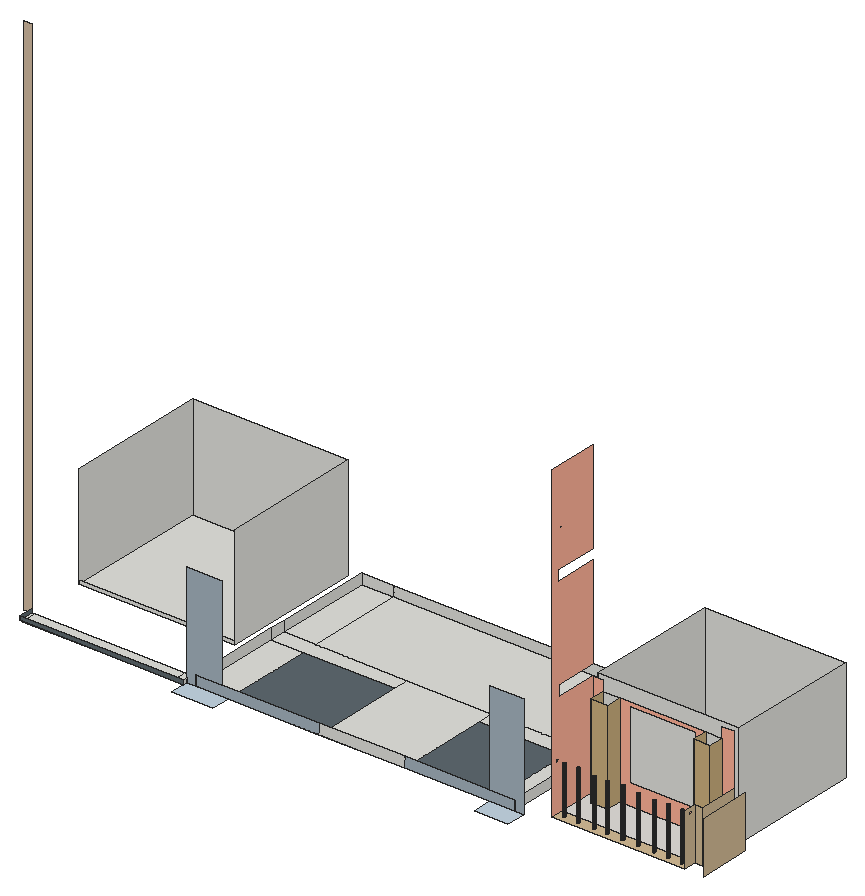
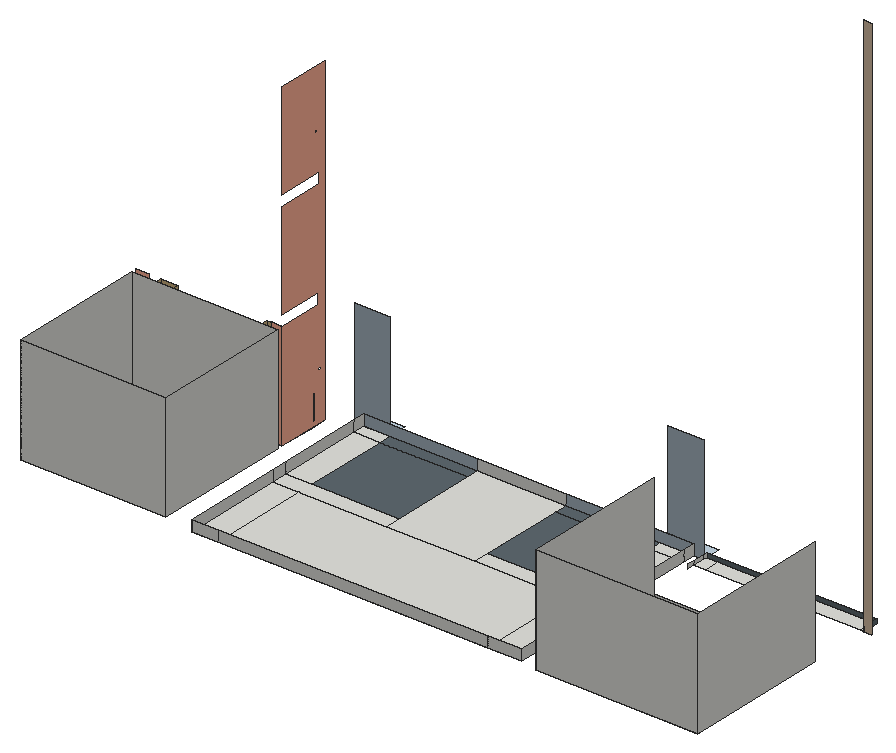
# SketchUp Ruby script. Lengths in inches.
U = 1.inch
M = Sketchup.active_model
def pt(a) = Geom::Point3d.new(a.map { |v| v * U })
def face(e, loops, mat)
  f = e.add_face(loops[0].map { |a| pt(a) })
  loops[1..].each { |l| e.add_face(l.map { |a| pt(a) }).erase! }
  f.material = f.back_material = mat if mat
  f
end
# faces: each face lists its corners as indices into pts; further lists are holes
def faces(e, pts, list, mat = nil) = list.each { |f| face(e, (f[0].is_a?(Array) ? f : [f]).map { |l| l.map { |i| pts[i] } }, mat) }
# xy, xz, yz: faces in a plane at the given z, y or x. An outline is a flat list of corners, or four numbers for a rectangle; further outlines are holes
def ring(l) = l.size == 4 ? [[l[0], l[1]], [l[2], l[1]], [l[2], l[3]], [l[0], l[3]]] : l.each_slice(2).to_a
def flat(e, list, mat, &to3) = list.each { |f| face(e, (f[0].is_a?(Array) ? f : [f]).map { |l| ring(l).map { |u, v| to3.(u, v) } }, mat) }
def xy(e, z, list, mat = nil) = flat(e, list, mat) { |x, y| [x, y, z] }
def xz(e, y, list, mat = nil) = flat(e, list, mat) { |x, z| [x, y, z] }
def yz(e, x, list, mat = nil) = flat(e, list, mat) { |y, z| [x, y, z] }
def lines(e, pts, list) = list.each { |a, b| e.add_line(pt(pts[a]), pt(pts[b])) }
# prism: a flat outline (further loops are holes) pulled along v
def prism(e, loops, v, mat = nil)
  f = face(e, loops, mat); d = Geom::Vector3d.new(v.map { |x| x * U })
  f.pushpull(f.normal.samedirection?(d) ? d.length : -d.length)
end
def box(e, o, s, mat = nil) = prism(e, [[o, [o[0] + s[0], o[1], o[2]], [o[0] + s[0], o[1] + s[1], o[2]], [o[0], o[1] + s[1], o[2]]]], [0, 0, s[2]], mat)
def at(x, y, z, deg = 0) = Geom::Transformation.translation(pt([x, y, z])) * Geom::Transformation.rotation(ORIGIN, Z_AXIS, deg.degrees)
def axes(o, x, y, z) = Geom::Transformation.new([*x, 0, *y, 0, *z, 0, *pt(o).to_a, 1])
def part(name) = M.definitions.add(name)
# library, detail: a bought-in or finely detailed component or shape, given as its bounding box
def library(name, o, s) = part(name).tap { |d| box(d.entities, o, s) }
def detail(e, o, s) = box(e.add_group.entities, o, s)
def put(e, d, t, mat = nil) = e.add_instance(d, t).tap { |i| i.material = mat if mat }
def group(e, t, mat = nil) = e.add_group.tap { |g| g.transformation = t; g.material = mat if mat }.entities
root = M.entities
M.materials.add("[Color B02]").color = [255, 178, 153]
M.materials.add("[Formica Beige]").color = [211, 187, 149]
M.materials.add("[Formica Laminate Dark]").color = [50, 53, 60]
M.materials.add("[Formica Laminate Light]").color = [213, 189, 164]
M.materials.add("[Formica Speckled Grey]").color = [94, 105, 111]
M.materials.add("[Terrazzo Light Blue]1").color = [165, 180, 191]
M.materials.add("[Terrazzo Light Blue]2").color = [196, 214, 227]
M.materials.add("[Terrazzo Tile Accent]").color = [224, 221, 217]
M.materials.add("[Wood Floor Light]").color = [204, 176, 127]
xy(root,129,[[9,105.54,12.72,122.79],[12.72,105.54,185.85,122.79],[185.85,105.54,198.57,122.79],[209,110.07,246.77,123.98],[351.88,110.07,450.54,237.1],
  [549.2,110.07,577.87,123.98],[209,123.98,246.77,219.13],[549.2,123.98,577.87,219.13],[619.39,128.83,619,128.89,618.64,129.04,618.33,129.27,618.09,129.58,617.9375,129.95,617.89,130.33,617.9375,130.72,618.09,131.08,618.33,131.4,618.64,131.63,619,131.78,619.39,131.83,619.78,131.78,620.14,131.63,620.45,131.4,620.6875,131.08,620.84,130.72,620.89,130.33,620.84,129.95,620.6875,129.58,620.45,129.27,620.14,129.04,619.78,128.89],[636.07,128.83,635.6875,128.89,635.32,129.04,635.01,129.27,634.78,129.58,634.625,129.95,634.57,130.33,634.625,130.72,634.78,131.08,635.01,131.4,635.32,131.63,635.6875,131.78,636.07,131.83,636.46,131.78,636.82,131.63,637.14,131.4,637.375,131.08,637.52,130.72,637.57,130.33,637.52,129.95,637.375,129.58,637.14,129.27,636.82,129.04,636.46,128.89],
  [654.01,128.83,653.625,128.89,653.26,129.04,652.95,129.27,652.71,129.58,652.5625,129.95,652.51,130.33,652.5625,130.72,652.71,131.08,652.95,131.4,653.26,131.63,653.625,131.78,654.01,131.83,654.4,131.78,654.76,131.63,655.07,131.4,655.3125,131.08,655.46,130.72,655.51,130.33,655.46,129.95,655.3125,129.58,655.07,129.27,654.76,129.04,654.4,128.89],[669.45,128.83,669.0625,128.89,668.7,129.04,668.39,129.27,668.15,129.58,668,129.95,667.95,130.33,668,130.72,668.15,131.08,668.39,131.4,668.7,131.63,669.0625,131.78,669.45,131.83,669.84,131.78,670.2,131.63,670.51,131.4,670.75,131.08,670.9,130.72,670.95,130.33,670.9,129.95,670.75,129.58,670.51,129.27,670.2,129.04,669.84,128.89],[687.39,128.83,687,128.89,686.64,129.04,686.33,129.27,686.09,129.58,685.9375,129.95,685.89,130.33,685.9375,130.72,686.09,131.08,686.33,131.4,686.64,131.63,687,131.78,687.39,131.83,687.78,131.78,688.14,131.63,688.45,131.4,688.6875,131.08,688.84,130.72,688.89,130.33,688.84,129.95,688.6875,129.58,688.45,129.27,688.14,129.04,687.78,128.89],[704.89,128.83,704.5,128.89,704.14,129.04,703.83,129.27,703.59,129.58,703.4375,129.95,703.39,130.33,703.4375,130.72,703.59,131.08,703.83,131.4,704.14,131.63,704.5,131.78,704.89,131.83,705.28,131.78,705.64,131.63,705.95,131.4,706.1875,131.08,706.34,130.72,706.39,130.33,706.34,129.95,706.1875,129.58,705.95,129.27,705.64,129.04,705.28,128.89],[723.39,128.83,723,128.89,722.64,129.04,722.33,129.27,722.09,129.58,721.9375,129.95,721.89,130.33,721.9375,130.72,722.09,131.08,722.33,131.4,722.64,131.63,723,131.78,723.39,131.83,723.78,131.78,724.14,131.63,724.45,131.4,724.6875,131.08,724.84,130.72,724.89,130.33,724.84,129.95,724.6875,129.58,724.45,129.27,724.14,129.04,723.78,128.89],
  [740.01,128.83,739.625,128.89,739.26,129.04,738.95,129.27,738.71,129.58,738.5625,129.95,738.51,130.33,738.5625,130.72,738.71,131.08,738.95,131.4,739.26,131.63,739.625,131.78,740.01,131.83,740.4,131.78,740.76,131.63,741.07,131.4,741.3125,131.08,741.46,130.72,741.51,130.33,741.46,129.95,741.3125,129.58,741.07,129.27,740.76,129.04,740.4,128.89],[756.14,128.83,755.75,128.89,755.39,129.04,755.08,129.27,754.84,129.58,754.6875,129.95,754.64,130.33,754.6875,130.72,754.84,131.08,755.08,131.4,755.39,131.63,755.75,131.78,756.14,131.83,756.53,131.78,756.89,131.63,757.2,131.4,757.4375,131.08,757.59,130.72,757.64,130.33,757.59,129.95,757.4375,129.58,757.2,129.27,756.89,129.04,756.53,128.89],[622.89,165.2,641.83,182.57],[741.45,165.2,760.39,182.57],[611.125,189.24,774.15,344.36],
  [9,191.15,189.57,355.125],[209,219.13,351.88,237.1],[450.54,219.13,577.87,237.1],[209,237.1,246.77,350.21],[246.77,237.1,549.2,350.21],
  [549.2,237.1,577.87,350.21]])
xy(root,129,[[[611.125,122.79,765.67,137.11],[619.39,128.83,619,128.89,618.64,129.04,618.33,129.27,618.09,129.58,617.9375,129.95,617.89,130.33,617.9375,130.72,618.09,131.08,618.33,131.4,618.64,131.63,619,131.78,619.39,131.83,619.78,131.78,620.14,131.63,620.45,131.4,620.6875,131.08,620.84,130.72,620.89,130.33,620.84,129.95,620.6875,129.58,620.45,129.27,620.14,129.04,619.78,128.89],[756.14,128.83,755.75,128.89,755.39,129.04,755.08,129.27,754.84,129.58,754.6875,129.95,754.64,130.33,754.6875,130.72,754.84,131.08,755.08,131.4,755.39,131.63,755.75,131.78,756.14,131.83,756.53,131.78,756.89,131.63,757.2,131.4,757.4375,131.08,757.59,130.72,757.64,130.33,757.59,129.95,757.4375,129.58,757.2,129.27,756.89,129.04,756.53,128.89],[636.07,128.83,635.6875,128.89,635.32,129.04,635.01,129.27,634.78,129.58,634.625,129.95,634.57,130.33,634.625,130.72,634.78,131.08,635.01,131.4,635.32,131.63,635.6875,131.78,636.07,131.83,636.46,131.78,636.82,131.63,637.14,131.4,637.375,131.08,637.52,130.72,637.57,130.33,637.52,129.95,637.375,129.58,637.14,129.27,636.82,129.04,636.46,128.89],[740.01,128.83,739.625,128.89,739.26,129.04,738.95,129.27,738.71,129.58,738.5625,129.95,738.51,130.33,738.5625,130.72,738.71,131.08,738.95,131.4,739.26,131.63,739.625,131.78,740.01,131.83,740.4,131.78,740.76,131.63,741.07,131.4,741.3125,131.08,741.46,130.72,741.51,130.33,741.46,129.95,741.3125,129.58,741.07,129.27,740.76,129.04,740.4,128.89],[654.01,128.83,653.625,128.89,653.26,129.04,652.95,129.27,652.71,129.58,652.5625,129.95,652.51,130.33,652.5625,130.72,652.71,131.08,652.95,131.4,653.26,131.63,653.625,131.78,654.01,131.83,654.4,131.78,654.76,131.63,655.07,131.4,655.3125,131.08,655.46,130.72,655.51,130.33,655.46,129.95,655.3125,129.58,655.07,129.27,654.76,129.04,654.4,128.89],[723.39,128.83,723,128.89,722.64,129.04,722.33,129.27,722.09,129.58,721.9375,129.95,721.89,130.33,721.9375,130.72,722.09,131.08,722.33,131.4,722.64,131.63,723,131.78,723.39,131.83,723.78,131.78,724.14,131.63,724.45,131.4,724.6875,131.08,724.84,130.72,724.89,130.33,724.84,129.95,724.6875,129.58,724.45,129.27,724.14,129.04,723.78,128.89],[669.45,128.83,669.0625,128.89,668.7,129.04,668.39,129.27,668.15,129.58,668,129.95,667.95,130.33,668,130.72,668.15,131.08,668.39,131.4,668.7,131.63,669.0625,131.78,669.45,131.83,669.84,131.78,670.2,131.63,670.51,131.4,670.75,131.08,670.9,130.72,670.95,130.33,670.9,129.95,670.75,129.58,670.51,129.27,670.2,129.04,669.84,128.89],[704.89,128.83,704.5,128.89,704.14,129.04,703.83,129.27,703.59,129.58,703.4375,129.95,703.39,130.33,703.4375,130.72,703.59,131.08,703.83,131.4,704.14,131.63,704.5,131.78,704.89,131.83,705.28,131.78,705.64,131.63,705.95,131.4,706.1875,131.08,706.34,130.72,706.39,130.33,706.34,129.95,706.1875,129.58,705.95,129.27,705.64,129.04,705.28,128.89],[687.39,128.83,687,128.89,686.64,129.04,686.33,129.27,686.09,129.58,685.9375,129.95,685.89,130.33,685.9375,130.72,686.09,131.08,686.33,131.4,686.64,131.63,687,131.78,687.39,131.83,687.78,131.78,688.14,131.63,688.45,131.4,688.6875,131.08,688.84,130.72,688.89,130.33,688.84,129.95,688.6875,129.58,688.45,129.27,688.14,129.04,687.78,128.89]]],"[Formica Beige]")
xy(root,129,[[246.77,110.07,351.88,123.98],[450.54,110.07,549.2,123.98],[246.77,123.98,351.88,219.13],[450.54,123.98,549.2,219.13]],"[Formica Speckled Grey]")
xy(root,129,[[198.57,88.2,246.77,110.07],[549.2,88.2,588.3,110.07]],"[Terrazzo Light Blue]2")
xy(root,129,[[611.125,137.11,774.15,137.11,774.15,182.57,760.39,182.57,760.39,165.2,741.45,165.2,741.45,182.57,641.83,182.57,641.83,165.2,622.89,165.2,622.89,182.57,611.125,182.57]],"[Terrazzo Tile Accent]")
xz(root,105.54,[[9,129,198.57,133.5625]],"[Formica Speckled Grey]")
xz(root,110.07,[[351.88,129,450.54,141]])
xz(root,110.07,[[198.57,129,209,129,209,141,238.58,141,238.58,249,198.57,249],[209,129,351.88,141],[450.54,129,577.87,141],[577.87,129,588.3,129,588.3,249,549.2,249,549.2,141,577.87,141]],"[Terrazzo Light Blue]1")
xz(root,122.79,[[0,129,9,740.5625]],"[Formica Laminate Light]")
xz(root,137.11,[[765.67,129,774.15,189]],"[Formica Beige]")
xz(root,165.2,[[622.89,129,641.83,236.59],[741.45,129,760.39,236.59]],"[Wood Floor Light]")
xz(root,182.57,[[622.89,129,641.83,236.59],[741.45,129,760.39,236.59]])
xz(root,182.57,[[611.125,129,622.89,249],[[641.83,129,741.45,236.59],[653.07,152.76,730.45,232.51]],[760.39,129,774.15,249]],"[Color B02]")
xz(root,189.24,[[611.125,129,774.15,249]])
xz(root,191.15,[[9,129,189.57,133.5625]])
xz(root,344.36,[[611.125,129,774.15,249]])
xz(root,350.21,[[209,129,246.77,141],[246.77,129,549.2,141],[549.2,129,577.87,141]])
xz(root,355.125,[[9,129,189.57,249]])
yz(root,9,[[191.15,129,355.125,249]])
yz(root,9,[[105.54,129,122.79,133.5625]],"[Formica Speckled Grey]")
yz(root,189.57,[[191.15,129,355.125,249]])
yz(root,198.57,[[105.54,129,110.07,133.5625],[110.07,129,122.79,133.5625],[122.79,129,131.79,133.5625]])
yz(root,209,[[110.07,129,123.98,141],[123.98,129,219.13,141],[219.13,129,237.1,141],[237.1,129,350.21,141]])
yz(root,577.87,[[110.07,129,123.98,141],[123.98,129,219.13,141],[219.13,129,237.1,141],[237.1,129,350.21,141]])
yz(root,611.125,[[189.24,129,344.36,249]])
yz(root,611.125,[[[122.79,129,182.57,129,182.57,249,133.3,249,133.3,261,182.57,261,182.57,369,131.74,369,131.74,381,182.57,381,182.57,489,122.79,489],[130.24,182.07,129.73,182.14,129.24,182.34,128.83,182.66,128.51,183.07,128.3125,183.55,128.24,184.07,128.3125,184.59,128.51,185.07,128.83,185.49,129.24,185.8,129.73,186,130.24,186.07,130.76,186,131.24,185.8,131.66,185.49,131.98,185.07,132.18,184.59,132.24,184.07,132.18,183.55,131.98,183.07,131.66,182.66,131.24,182.34,130.76,182.14],[135.46,422.23,135.01,422.29,134.58,422.46,134.22,422.74,133.94,423.1,133.77,423.53,133.71,423.98,133.77,424.43,133.94,424.85,134.22,425.22,134.58,425.49,135.01,425.67,135.46,425.73,135.91,425.67,136.33,425.49,136.7,425.22,136.98,424.85,137.15,424.43,137.21,423.98,137.15,423.53,136.98,423.1,136.7,422.74,136.33,422.46,135.91,422.29],[138.08,300.72,137.78,300.77,137.49,300.88,137.25,301.07,137.06,301.32,136.9375,301.6,136.9,301.91,136.9375,302.22,137.06,302.51,137.25,302.75,137.49,302.94,137.78,303.06,138.08,303.1,138.39,303.06,138.68,302.94,138.92,302.75,139.11,302.51,139.23,302.22,139.27,301.91,139.23,301.6,139.11,301.32,138.92,301.07,138.68,300.88,138.39,300.77]]],"[Color B02]")
yz(root,622.89,[[165.2,129,182.57,236.59]],"[Wood Floor Light]")
yz(root,641.83,[[165.2,129,182.57,236.59]],"[Wood Floor Light]")
yz(root,741.45,[[165.2,129,182.57,236.59]],"[Wood Floor Light]")
yz(root,760.39,[[165.2,129,182.57,236.59]],"[Wood Floor Light]")
yz(root,765.67,[[[122.79,129,137.11,189],[130.24,182.07,130.76,182.14,131.24,182.34,131.66,182.66,131.98,183.07,132.18,183.55,132.24,184.07,132.18,184.59,131.98,185.07,131.66,185.49,131.24,185.8,130.76,186,130.24,186.07,129.73,186,129.24,185.8,128.83,185.49,128.51,185.07,128.3125,184.59,128.24,184.07,128.3125,183.55,128.51,183.07,128.83,182.66,129.24,182.34,129.73,182.14]]],"[Formica Beige]")
yz(root,774.15,[[189.24,129,344.36,249]])
yz(root,774.15,[[137.11,129,182.57,189]],"[Formica Beige]")
yz(root,786.87,[[122.79,129,182.57,189]],"[Formica Beige]")
p = [[619,128.89,129],[619.39,128.83,129],[619.39,128.83,184.1875],[619,128.89,184.1875],[619.78,128.89,129],[619.78,128.89,184.1875],
  [635.6875,128.89,129],[636.07,128.83,129],[636.07,128.83,185.07],[635.6875,128.89,185.07],[636.46,128.89,129],[636.46,128.89,185.07],
  [653.625,128.89,129],[654.01,128.83,129],[654.01,128.83,182.75],[653.625,128.89,182.75],[654.4,128.89,129],[654.4,128.89,182.75],
  [669.0625,128.89,129],[669.45,128.83,129],[669.45,128.83,182.9375],[669.0625,128.89,182.9375],[669.84,128.89,129],[669.84,128.89,182.9375],
  [687,128.89,129],[687.39,128.83,129],[687.39,128.83,185.07],[687,128.89,185.07],[687.78,128.89,129],[687.78,128.89,185.07],
  [704.5,128.89,129],[704.89,128.83,129],[704.89,128.83,183.1875],[704.5,128.89,183.1875],[705.28,128.89,129],[705.28,128.89,183.1875],
  [723,128.89,129],[723.39,128.83,129],[723.39,128.83,182],[723,128.89,182],[723.78,128.89,129],[723.78,128.89,182],
  [739.625,128.89,129],[740.01,128.83,129],[740.01,128.83,183.5625],[739.625,128.89,183.5625],[740.4,128.89,129],[740.4,128.89,183.5625],
  [755.75,128.89,129],[756.14,128.83,129],[756.14,128.83,183.5625],[755.75,128.89,183.5625],[756.53,128.89,129],[756.53,128.89,183.5625],
  [618.64,129.04,129],[618.64,129.04,184.1875],[620.14,129.04,129],[620.14,129.04,184.1875],[635.32,129.04,129],[635.32,129.04,185.07],
  [636.82,129.04,129],[636.82,129.04,185.07],[653.26,129.04,129],[653.26,129.04,182.75],[654.76,129.04,129],[654.76,129.04,182.75],
  [668.7,129.04,129],[668.7,129.04,182.9375],[670.2,129.04,129],[670.2,129.04,182.9375],[686.64,129.04,129],[686.64,129.04,185.07],
  [688.14,129.04,129],[688.14,129.04,185.07],[704.14,129.04,129],[704.14,129.04,183.1875],[705.64,129.04,129],[705.64,129.04,183.1875],
  [722.64,129.04,129],[722.64,129.04,182],[724.14,129.04,129],[724.14,129.04,182],[739.26,129.04,129],[739.26,129.04,183.5625],
  [740.76,129.04,129],[740.76,129.04,183.5625],[755.39,129.04,129],[755.39,129.04,183.5625],[756.89,129.04,129],[756.89,129.04,183.5625],
  [618.33,129.27,129],[618.33,129.27,184.1875],[620.45,129.27,129],[620.45,129.27,184.1875],[635.01,129.27,129],[635.01,129.27,185.07],
  [637.14,129.27,129],[637.14,129.27,185.07],[652.95,129.27,129],[652.95,129.27,182.75],[655.07,129.27,129],[655.07,129.27,182.75],
  [668.39,129.27,129],[668.39,129.27,182.9375],[670.51,129.27,129],[670.51,129.27,182.9375],[686.33,129.27,129],[686.33,129.27,185.07],
  [688.45,129.27,129],[688.45,129.27,185.07],[703.83,129.27,129],[703.83,129.27,183.1875],[705.95,129.27,129],[705.95,129.27,183.1875],
  [722.33,129.27,129],[722.33,129.27,182],[724.45,129.27,129],[724.45,129.27,182],[738.95,129.27,129],[738.95,129.27,183.5625],
  [741.07,129.27,129],[741.07,129.27,183.5625],[755.08,129.27,129],[755.08,129.27,183.5625],[757.2,129.27,129],[757.2,129.27,183.5625],
  [618.09,129.58,129],[618.09,129.58,184.1875],[620.6875,129.58,129],[620.6875,129.58,184.1875],[634.78,129.58,129],[634.78,129.58,185.07],
  [637.375,129.58,129],[637.375,129.58,185.07],[652.71,129.58,129],[652.71,129.58,182.75],[655.3125,129.58,129],[655.3125,129.58,182.75],
  [668.15,129.58,129],[668.15,129.58,182.9375],[670.75,129.58,129],[670.75,129.58,182.9375],[686.09,129.58,129],[686.09,129.58,185.07],
  [688.6875,129.58,129],[688.6875,129.58,185.07],[703.59,129.58,129],[703.59,129.58,183.1875],[706.1875,129.58,129],[706.1875,129.58,183.1875],
  [722.09,129.58,129],[722.09,129.58,182],[724.6875,129.58,129],[724.6875,129.58,182],[738.71,129.58,129],[738.71,129.58,183.5625],
  [741.3125,129.58,129],[741.3125,129.58,183.5625],[754.84,129.58,129],[754.84,129.58,183.5625],[757.4375,129.58,129],[757.4375,129.58,183.5625],
  [617.9375,129.95,129],[617.9375,129.95,184.1875],[620.84,129.95,129],[620.84,129.95,184.1875],[634.625,129.95,129],[634.625,129.95,185.07],
  [637.52,129.95,129],[637.52,129.95,185.07],[652.5625,129.95,129],[652.5625,129.95,182.75],[655.46,129.95,129],[655.46,129.95,182.75],
  [668,129.95,129],[668,129.95,182.9375],[670.9,129.95,129],[670.9,129.95,182.9375],[685.9375,129.95,129],[685.9375,129.95,185.07],
  [688.84,129.95,129],[688.84,129.95,185.07],[703.4375,129.95,129],[703.4375,129.95,183.1875],[706.34,129.95,129],[706.34,129.95,183.1875],
  [721.9375,129.95,129],[721.9375,129.95,182],[724.84,129.95,129],[724.84,129.95,182],[738.5625,129.95,129],[738.5625,129.95,183.5625],
  [741.46,129.95,129],[741.46,129.95,183.5625],[754.6875,129.95,129],[754.6875,129.95,183.5625],[757.59,129.95,129],[757.59,129.95,183.5625],
  [617.89,130.33,129],[617.89,130.33,184.1875],[620.89,130.33,129],[620.89,130.33,184.1875],[634.57,130.33,129],[634.57,130.33,185.07],
  [637.57,130.33,129],[637.57,130.33,185.07],[652.51,130.33,129],[652.51,130.33,182.75],[655.51,130.33,129],[655.51,130.33,182.75],
  [667.95,130.33,129],[667.95,130.33,182.9375],[670.95,130.33,129],[670.95,130.33,182.9375],[685.89,130.33,129],[685.89,130.33,185.07],
  [688.89,130.33,129],[688.89,130.33,185.07],[703.39,130.33,129],[703.39,130.33,183.1875],[706.39,130.33,129],[706.39,130.33,183.1875],
  [721.89,130.33,129],[721.89,130.33,182],[724.89,130.33,129],[724.89,130.33,182],[738.51,130.33,129],[738.51,130.33,183.5625],
  [741.51,130.33,129],[741.51,130.33,183.5625],[754.64,130.33,129],[754.64,130.33,183.5625],[757.64,130.33,129],[757.64,130.33,183.5625],
  [617.9375,130.72,129],[617.9375,130.72,184.1875],[620.84,130.72,129],[620.84,130.72,184.1875],[634.625,130.72,129],[634.625,130.72,185.07],
  [637.52,130.72,129],[637.52,130.72,185.07],[652.5625,130.72,129],[652.5625,130.72,182.75],[655.46,130.72,129],[655.46,130.72,182.75],
  [668,130.72,129],[668,130.72,182.9375],[670.9,130.72,129],[670.9,130.72,182.9375],[685.9375,130.72,129],[685.9375,130.72,185.07],
  [688.84,130.72,129],[688.84,130.72,185.07],[703.4375,130.72,129],[703.4375,130.72,183.1875],[706.34,130.72,129],[706.34,130.72,183.1875],
  [721.9375,130.72,129],[721.9375,130.72,182],[724.84,130.72,129],[724.84,130.72,182],[738.5625,130.72,129],[738.5625,130.72,183.5625],
  [741.46,130.72,129],[741.46,130.72,183.5625],[754.6875,130.72,129],[754.6875,130.72,183.5625],[757.59,130.72,129],[757.59,130.72,183.5625],
  [618.09,131.08,129],[618.09,131.08,184.1875],[620.6875,131.08,129],[620.6875,131.08,184.1875],[634.78,131.08,129],[634.78,131.08,185.07],
  [637.375,131.08,129],[637.375,131.08,185.07],[652.71,131.08,129],[652.71,131.08,182.75],[655.3125,131.08,129],[655.3125,131.08,182.75],
  [668.15,131.08,129],[668.15,131.08,182.9375],[670.75,131.08,129],[670.75,131.08,182.9375],[686.09,131.08,129],[686.09,131.08,185.07],
  [688.6875,131.08,129],[688.6875,131.08,185.07],[703.59,131.08,129],[703.59,131.08,183.1875],[706.1875,131.08,129],[706.1875,131.08,183.1875],
  [722.09,131.08,129],[722.09,131.08,182],[724.6875,131.08,129],[724.6875,131.08,182],[738.71,131.08,129],[738.71,131.08,183.5625],
  [741.3125,131.08,129],[741.3125,131.08,183.5625],[754.84,131.08,129],[754.84,131.08,183.5625],[757.4375,131.08,129],[757.4375,131.08,183.5625],
  [618.33,131.4,129],[618.33,131.4,184.1875],[620.45,131.4,129],[620.45,131.4,184.1875],[635.01,131.4,129],[635.01,131.4,185.07],
  [637.14,131.4,129],[637.14,131.4,185.07],[652.95,131.4,129],[652.95,131.4,182.75],[655.07,131.4,129],[655.07,131.4,182.75],
  [668.39,131.4,129],[668.39,131.4,182.9375],[670.51,131.4,129],[670.51,131.4,182.9375],[686.33,131.4,129],[686.33,131.4,185.07],
  [688.45,131.4,129],[688.45,131.4,185.07],[703.83,131.4,129],[703.83,131.4,183.1875],[705.95,131.4,129],[705.95,131.4,183.1875],
  [722.33,131.4,129],[722.33,131.4,182],[724.45,131.4,129],[724.45,131.4,182],[738.95,131.4,129],[738.95,131.4,183.5625],
  [741.07,131.4,129],[741.07,131.4,183.5625],[755.08,131.4,129],[755.08,131.4,183.5625],[757.2,131.4,129],[757.2,131.4,183.5625],
  [618.64,131.63,129],[618.64,131.63,184.1875],[620.14,131.63,129],[620.14,131.63,184.1875],[635.32,131.63,129],[635.32,131.63,185.07],
  [636.82,131.63,129],[636.82,131.63,185.07],[653.26,131.63,129],[653.26,131.63,182.75],[654.76,131.63,129],[654.76,131.63,182.75],
  [668.7,131.63,129],[668.7,131.63,182.9375],[670.2,131.63,129],[670.2,131.63,182.9375],[686.64,131.63,129],[686.64,131.63,185.07],
  [688.14,131.63,129],[688.14,131.63,185.07],[704.14,131.63,129],[704.14,131.63,183.1875],[705.64,131.63,129],[705.64,131.63,183.1875],
  [722.64,131.63,129],[722.64,131.63,182],[724.14,131.63,129],[724.14,131.63,182],[739.26,131.63,129],[739.26,131.63,183.5625],
  [740.76,131.63,129],[740.76,131.63,183.5625],[755.39,131.63,129],[755.39,131.63,183.5625],[756.89,131.63,129],[756.89,131.63,183.5625],
  [619,131.78,129],[619,131.78,184.1875],[619.78,131.78,129],[619.78,131.78,184.1875],[635.6875,131.78,129],[635.6875,131.78,185.07],
  [636.46,131.78,129],[636.46,131.78,185.07],[653.625,131.78,129],[653.625,131.78,182.75],[654.4,131.78,129],[654.4,131.78,182.75],
  [669.0625,131.78,129],[669.0625,131.78,182.9375],[669.84,131.78,129],[669.84,131.78,182.9375],[687,131.78,129],[687,131.78,185.07],
  [687.78,131.78,129],[687.78,131.78,185.07],[704.5,131.78,129],[704.5,131.78,183.1875],[705.28,131.78,129],[705.28,131.78,183.1875],
  [723,131.78,129],[723,131.78,182],[723.78,131.78,129],[723.78,131.78,182],[739.625,131.78,129],[739.625,131.78,183.5625],
  [740.4,131.78,129],[740.4,131.78,183.5625],[755.75,131.78,129],[755.75,131.78,183.5625],[756.53,131.78,129],[756.53,131.78,183.5625],
  [619.39,131.83,129],[619.39,131.83,184.1875],[636.07,131.83,129],[636.07,131.83,185.07],[654.01,131.83,129],[654.01,131.83,182.75],
  [669.45,131.83,129],[669.45,131.83,182.9375],[687.39,131.83,129],[687.39,131.83,185.07],[704.89,131.83,129],[704.89,131.83,183.1875],
  [723.39,131.83,129],[723.39,131.83,182],[740.01,131.83,129],[740.01,131.83,183.5625],[756.14,131.83,129],[756.14,131.83,183.5625]]
faces(root,p,[[0,1,2,3],[1,4,5,2],[6,7,8,9],[7,10,11,8],[12,13,14,15],[13,16,17,14],[18,19,20,21],[19,22,23,20],
  [24,25,26,27],[25,28,29,26],[30,31,32,33],[31,34,35,32],[36,37,38,39],[37,40,41,38],[42,43,44,45],[43,46,47,44],
  [48,49,50,51],[49,52,53,50],[54,0,3,55],[4,56,57,5],[58,6,9,59],[10,60,61,11],[62,12,15,63],[16,64,65,17],
  [66,18,21,67],[22,68,69,23],[70,24,27,71],[28,72,73,29],[74,30,33,75],[34,76,77,35],[78,36,39,79],[40,80,81,41],
  [82,42,45,83],[46,84,85,47],[86,48,51,87],[52,88,89,53],[90,54,55,91],[56,92,93,57],[94,58,59,95],[60,96,97,61],
  [98,62,63,99],[64,100,101,65],[102,66,67,103],[68,104,105,69],[106,70,71,107],[72,108,109,73],[110,74,75,111],[76,112,113,77],
  [114,78,79,115],[80,116,117,81],[118,82,83,119],[84,120,121,85],[122,86,87,123],[88,124,125,89],[126,90,91,127],[92,128,129,93],
  [130,94,95,131],[96,132,133,97],[134,98,99,135],[100,136,137,101],[138,102,103,139],[104,140,141,105],[142,106,107,143],[108,144,145,109],
  [146,110,111,147],[112,148,149,113],[150,114,115,151],[116,152,153,117],[154,118,119,155],[120,156,157,121],[158,122,123,159],[124,160,161,125],
  [162,126,127,163],[128,164,165,129],[166,130,131,167],[132,168,169,133],[170,134,135,171],[136,172,173,137],[174,138,139,175],[140,176,177,141],
  [178,142,143,179],[144,180,181,145],[182,146,147,183],[148,184,185,149],[186,150,151,187],[152,188,189,153],[190,154,155,191],[156,192,193,157],
  [194,158,159,195],[160,196,197,161],[198,162,163,199],[164,200,201,165],[202,166,167,203],[168,204,205,169],[206,170,171,207],[172,208,209,173],
  [210,174,175,211],[176,212,213,177],[214,178,179,215],[180,216,217,181],[218,182,183,219],[184,220,221,185],[222,186,187,223],[188,224,225,189],
  [226,190,191,227],[192,228,229,193],[230,194,195,231],[196,232,233,197],[234,198,199,235],[200,236,237,201],[238,202,203,239],[204,240,241,205],
  [242,206,207,243],[208,244,245,209],[246,210,211,247],[212,248,249,213],[250,214,215,251],[216,252,253,217],[254,218,219,255],[220,256,257,221],
  [258,222,223,259],[224,260,261,225],[262,226,227,263],[228,264,265,229],[266,230,231,267],[232,268,269,233],[270,234,235,271],[236,272,273,237],
  [274,238,239,275],[240,276,277,241],[278,242,243,279],[244,280,281,245],[282,246,247,283],[248,284,285,249],[286,250,251,287],[252,288,289,253],
  [290,254,255,291],[256,292,293,257],[294,258,259,295],[260,296,297,261],[298,262,263,299],[264,300,301,265],[302,266,267,303],[268,304,305,269],
  [306,270,271,307],[272,308,309,273],[310,274,275,311],[276,312,313,277],[314,278,279,315],[280,316,317,281],[318,282,283,319],[284,320,321,285],
  [322,286,287,323],[288,324,325,289],[326,290,291,327],[292,328,329,293],[330,294,295,331],[296,332,333,297],[334,298,299,335],[300,336,337,301],
  [338,302,303,339],[304,340,341,305],[342,306,307,343],[308,344,345,309],[346,310,311,347],[312,348,349,313],[350,314,315,351],[316,352,353,317],
  [354,318,319,355],[320,356,357,321],[358,322,323,359],[324,360,361,325],[362,326,327,363],[328,364,365,329],[366,330,331,367],[332,368,369,333],
  [370,334,335,371],[336,372,373,337],[374,338,339,375],[340,376,377,341],[378,342,343,379],[344,380,381,345],[382,346,347,383],[348,384,385,349],
  [386,350,351,387],[352,388,389,353],[390,354,355,391],[356,392,393,357],[394,358,359,395],[360,396,397,361],[398,362,363,399],[364,400,401,365],
  [402,366,367,403],[368,404,405,369],[406,370,371,407],[372,408,409,373],[410,374,375,411],[376,412,413,377],[414,378,379,415],[380,414,415,381],
  [416,382,383,417],[384,416,417,385],[418,386,387,419],[388,418,419,389],[420,390,391,421],[392,420,421,393],[422,394,395,423],[396,422,423,397],
  [424,398,399,425],[400,424,425,401],[426,402,403,427],[404,426,427,405],[428,406,407,429],[408,428,429,409],[430,410,411,431],[412,430,431,413]],"[Formica Laminate Dark]")
